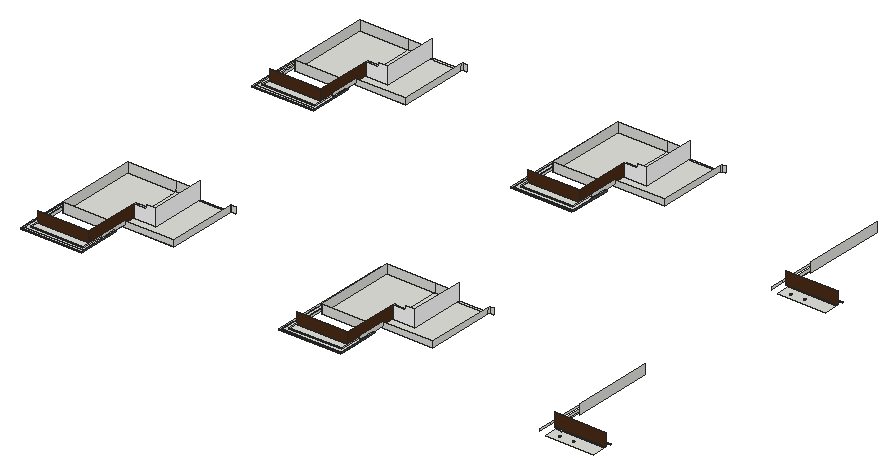
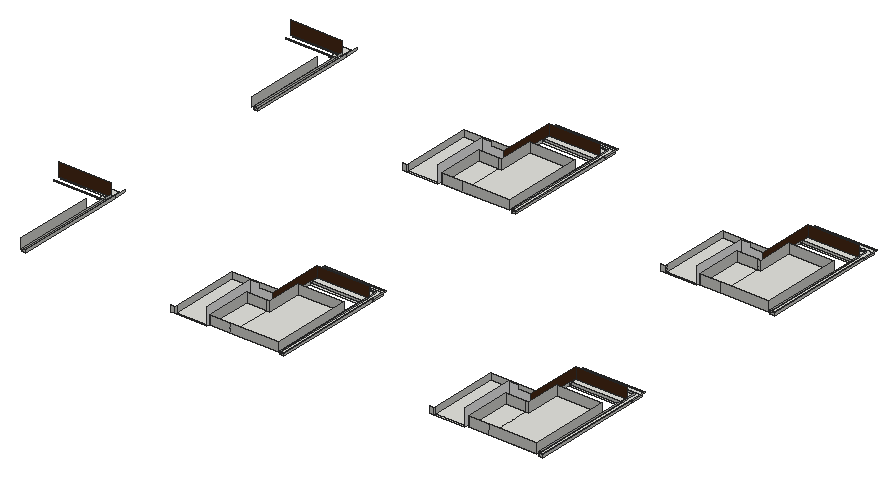
# SketchUp Ruby script. Lengths in inches.
U = 1.inch
M = Sketchup.active_model
def pt(a) = Geom::Point3d.new(a.map { |v| v * U })
def face(e, loops, mat)
  f = e.add_face(loops[0].map { |a| pt(a) })
  loops[1..].each { |l| e.add_face(l.map { |a| pt(a) }).erase! }
  f.material = f.back_material = mat if mat
  f
end
# faces: each face lists its corners as indices into pts; further lists are holes
def faces(e, pts, list, mat = nil) = list.each { |f| face(e, (f[0].is_a?(Array) ? f : [f]).map { |l| l.map { |i| pts[i] } }, mat) }
# xy, xz, yz: faces in a plane at the given z, y or x. An outline is a flat list of corners, or four numbers for a rectangle; further outlines are holes
def ring(l) = l.size == 4 ? [[l[0], l[1]], [l[2], l[1]], [l[2], l[3]], [l[0], l[3]]] : l.each_slice(2).to_a
def flat(e, list, mat, &to3) = list.each { |f| face(e, (f[0].is_a?(Array) ? f : [f]).map { |l| ring(l).map { |u, v| to3.(u, v) } }, mat) }
def xy(e, z, list, mat = nil) = flat(e, list, mat) { |x, y| [x, y, z] }
def xz(e, y, list, mat = nil) = flat(e, list, mat) { |x, z| [x, y, z] }
def yz(e, x, list, mat = nil) = flat(e, list, mat) { |y, z| [x, y, z] }
def lines(e, pts, list) = list.each { |a, b| e.add_line(pt(pts[a]), pt(pts[b])) }
# prism: a flat outline (further loops are holes) pulled along v
def prism(e, loops, v, mat = nil)
  f = face(e, loops, mat); d = Geom::Vector3d.new(v.map { |x| x * U })
  f.pushpull(f.normal.samedirection?(d) ? d.length : -d.length)
end
def box(e, o, s, mat = nil) = prism(e, [[o, [o[0] + s[0], o[1], o[2]], [o[0] + s[0], o[1] + s[1], o[2]], [o[0], o[1] + s[1], o[2]]]], [0, 0, s[2]], mat)
def at(x, y, z, deg = 0) = Geom::Transformation.translation(pt([x, y, z])) * Geom::Transformation.rotation(ORIGIN, Z_AXIS, deg.degrees)
def axes(o, x, y, z) = Geom::Transformation.new([*x, 0, *y, 0, *z, 0, *pt(o).to_a, 1])
def part(name) = M.definitions.add(name)
# library, detail: a bought-in or finely detailed component or shape, given as its bounding box
def library(name, o, s) = part(name).tap { |d| box(d.entities, o, s) }
def detail(e, o, s) = box(e.add_group.entities, o, s)
def put(e, d, t, mat = nil) = e.add_instance(d, t).tap { |i| i.material = mat if mat }
def group(e, t, mat = nil) = e.add_group.tap { |g| g.transformation = t; g.material = mat if mat }.entities
root = M.entities
M.materials.add("[Color M00]").color = [255, 255, 255]
M.materials.add("[Color M06]").color = [86, 86, 86]
M.materials.add("[Wood Veneer 01]").color = [76, 44, 23]
xy(root,257.1875,[[[2084.76,592.75,2251.32,636.6875],[2116.33,609.37,2117.03,609.46,2117.68,609.73,2118.23,610.15,2118.66,610.71,2118.93,611.36,2119.02,612.06,2118.93,612.75,2118.66,613.4,2118.23,613.96,2117.68,614.38,2117.03,614.65,2116.33,614.74,2115.64,614.65,2114.99,614.38,2114.43,613.96,2114.01,613.4,2113.74,612.75,2113.65,612.06,2113.74,611.36,2114.01,610.71,2114.43,610.15,2114.99,609.73,2115.64,609.46],[2164.33,609.37,2165.03,609.46,2165.68,609.73,2166.23,610.15,2166.66,610.71,2166.93,611.36,2167.02,612.06,2166.93,612.75,2166.66,613.4,2166.23,613.96,2165.68,614.38,2165.03,614.65,2164.33,614.74,2163.64,614.65,2162.99,614.38,2162.43,613.96,2162.01,613.4,2161.74,612.75,2161.65,612.06,2161.74,611.36,2162.01,610.71,2162.43,610.15,2162.99,609.73,2163.64,609.46],[2228.96,609.37,2229.65,609.46,2230.3,609.73,2230.86,610.15,2231.29,610.71,2231.55,611.36,2231.65,612.06,2231.55,612.75,2231.29,613.4,2230.86,613.96,2230.3,614.38,2229.65,614.65,2228.96,614.74,2228.26,614.65,2227.61,614.38,2227.06,613.96,2226.63,613.4,2226.36,612.75,2226.27,612.06,2226.36,611.36,2226.63,610.71,2227.06,610.15,2227.61,609.73,2228.26,609.46]],[2094.14,636.6875,2106.51,660.21],[[2084.76,1592.1,2251.32,1636.04],[2116.33,1608.72,2117.03,1608.8125,2117.68,1609.08,2118.23,1609.51,2118.66,1610.07,2118.93,1610.71,2119.02,1611.41,2118.93,1612.11,2118.66,1612.75,2118.23,1613.3125,2117.68,1613.74,2117.03,1614.01,2116.33,1614.1,2115.64,1614.01,2114.99,1613.74,2114.43,1613.3125,2114.01,1612.75,2113.74,1612.11,2113.65,1611.41,2113.74,1610.71,2114.01,1610.07,2114.43,1609.51,2114.99,1609.08,2115.64,1608.8125],[2164.33,1608.72,2165.03,1608.8125,2165.68,1609.08,2166.23,1609.51,2166.66,1610.07,2166.93,1610.71,2167.02,1611.41,2166.93,1612.11,2166.66,1612.75,2166.23,1613.3125,2165.68,1613.74,2165.03,1614.01,2164.33,1614.1,2163.64,1614.01,2162.99,1613.74,2162.43,1613.3125,2162.01,1612.75,2161.74,1612.11,2161.65,1611.41,2161.74,1610.71,2162.01,1610.07,2162.43,1609.51,2162.99,1609.08,2163.64,1608.8125],[2228.96,1608.72,2229.65,1608.8125,2230.3,1609.08,2230.86,1609.51,2231.29,1610.07,2231.55,1610.71,2231.65,1611.41,2231.55,1612.11,2231.29,1612.75,2230.86,1613.3125,2230.3,1613.74,2229.65,1614.01,2228.96,1614.1,2228.26,1614.01,2227.61,1613.74,2227.06,1613.3125,2226.63,1612.75,2226.36,1612.11,2226.27,1611.41,2226.36,1610.71,2226.63,1610.07,2227.06,1609.51,2227.61,1609.08,2228.26,1608.8125]],[2094.14,1636.04,2106.51,1659.57]])
xy(root,258.1875,[[294.47,639.17,471.68,662.52],[1187.0625,639.17,1364.27,662.52],[294.47,662.52,471.68,670.48],[1187.0625,662.52,1364.27,670.48],[304.78,733.75,462.15,733.75,462.15,854.49,471.68,854.49,471.68,1014.93,304.78,1014.93],
  [1197.375,733.75,1354.74,733.75,1354.74,854.49,1364.27,854.49,1364.27,1014.93,1197.375,1014.93],[471.68,776.62,655.66,776.62,655.66,1014.93,548.11,1014.93,548.11,832.12,471.68,832.12],[1364.27,776.62,1548.25,776.62,1548.25,1014.93,1440.7,1014.93,1440.7,832.12,1364.27,832.12],[471.68,854.49,542.11,1014.93],[1364.27,854.49,1434.7,1014.93],
  [548.11,1014.93,655.66,1021.31],[1440.7,1014.93,1548.25,1021.31],[294.47,1638.53,471.68,1661.875],[1187.0625,1638.53,1364.27,1661.875],[294.47,1661.875,471.68,1669.84],
  [1187.0625,1661.875,1364.27,1669.84],[304.78,1733.11,462.15,1733.11,462.15,1853.85,471.68,1853.85,471.68,2014.29,304.78,2014.29],[1197.375,1733.11,1354.74,1733.11,1354.74,1853.85,1364.27,1853.85,1364.27,2014.29,1197.375,2014.29],[471.68,1775.97,655.66,1775.97,655.66,2014.29,548.11,2014.29,548.11,1831.47,471.68,1831.47],[1364.27,1775.97,1548.25,1775.97,1548.25,2014.29,1440.7,2014.29,1440.7,1831.47,1364.27,1831.47],
  [471.68,1853.85,542.11,2014.29],[1364.27,1853.85,1434.7,2014.29],[548.11,2014.29,655.66,2020.66],[1440.7,2014.29,1548.25,2020.66]])
xy(root,265.6875,[[278.36,584.06,490.8,595.06],[1170.95,584.06,1383.39,595.06],[278.36,595.06,279.74,638.99],[279.74,595.06,279.74,1021.31,294.47,1021.31,294.47,607.33,475.29,607.33,475.29,706.17,484.3,706.17,484.3,595.06],[484.3,595.06,490.8,638.99],
  [1170.95,595.06,1172.33,638.99],[1172.33,595.06,1172.33,1021.31,1187.0625,1021.31,1187.0625,607.33,1367.875,607.33,1367.875,706.17,1376.89,706.17,1376.89,595.06],[1376.89,595.06,1383.39,638.99],[294.47,607.33,475.29,607.33,475.29,706.17,471.68,706.17,471.68,662.52,294.47,662.52],[1187.0625,607.33,1367.875,607.33,1367.875,706.17,1364.27,706.17,1364.27,662.52,1187.0625,662.52],
  [484.3,638.99,490.8,731.24],[1376.89,638.99,1383.39,731.24],[471.68,706.17,484.3,776.62],[1364.27,706.17,1376.89,776.62],[278.36,1583.41,490.8,1594.41],
  [1170.95,1583.41,1383.39,1594.41],[278.36,1594.41,279.74,1638.35],[279.74,1594.41,279.74,2020.66,294.47,2020.66,294.47,1606.6875,475.29,1606.6875,475.29,1705.53,484.3,1705.53,484.3,1594.41],[484.3,1594.41,490.8,1638.35],[1170.95,1594.41,1172.33,1638.35],
  [1172.33,1594.41,1172.33,2020.66,1187.0625,2020.66,1187.0625,1606.6875,1367.875,1606.6875,1367.875,1705.53,1376.89,1705.53,1376.89,1594.41],[1376.89,1594.41,1383.39,1638.35],[294.47,1606.6875,475.29,1606.6875,475.29,1705.53,471.68,1705.53,471.68,1661.875,294.47,1661.875],[1187.0625,1606.6875,1367.875,1606.6875,1367.875,1705.53,1364.27,1705.53,1364.27,1661.875,1187.0625,1661.875],[484.3,1638.35,490.8,1730.6],
  [1376.89,1638.35,1383.39,1730.6],[471.68,1705.53,484.3,1775.97],[1364.27,1705.53,1376.89,1775.97]])
xz(root,584.06,[[278.36,265.6875,490.8,269.375],[1170.95,265.6875,1383.39,269.375]],"[Color M06]")
xz(root,607.33,[[294.47,265.6875,475.29,269.375],[1187.0625,265.6875,1367.875,269.375]])
xz(root,636.86,[[2079.65,262.875,2256.86,307.5]],"[Wood Veneer 01]")
xz(root,638.99,[[278.36,265.6875,279.74,269.375],[1170.95,265.6875,1172.33,269.375]])
xz(root,639.17,[[294.47,258.1875,471.68,302.8125],[1187.0625,258.1875,1364.27,302.8125]],"[Wood Veneer 01]")
xz(root,660.21,[[2079.65,259.3125,2256.86,262.875]])
xz(root,662.52,[[294.47,258.1875,471.68,265.6875],[1187.0625,258.1875,1364.27,265.6875]])
xz(root,706.17,[[475.29,265.6875,484.3,269.375],[1367.875,265.6875,1376.89,269.375]])
xz(root,733.75,[[304.78,258.1875,462.15,291.125],[1197.375,258.1875,1354.74,291.125]])
xz(root,776.62,[[471.68,258.1875,471.68,265.6875,484.3,265.6875,484.3,279.25,655.66,279.25,655.66,258.1875],[1364.27,258.1875,1364.27,265.6875,1376.89,265.6875,1376.89,279.25,1548.25,279.25,1548.25,258.1875]])
xz(root,832.12,[[471.68,258.1875,548.11,258.1875,548.11,316.0625,518.11,316.0625,518.11,302.8125,471.68,302.8125],[1364.27,258.1875,1440.7,258.1875,1440.7,316.0625,1410.7,316.0625,1410.7,302.8125,1364.27,302.8125]],"[Color M00]")
xz(root,854.49,[[462.15,258.1875,471.68,291.125],[471.68,258.1875,542.11,291.125],[1354.74,258.1875,1364.27,291.125],[1364.27,258.1875,1434.7,291.125]])
xz(root,1014.93,[[304.78,258.1875,471.68,291.125],[471.68,258.1875,542.11,291.125],[1197.375,258.1875,1364.27,291.125],[1364.27,258.1875,1434.7,291.125]])
xz(root,1019,[[2064.92,262.875,2079.65,270.375]])
xz(root,1021.31,[[279.74,258.1875,294.47,265.6875],[655.66,258.1875,671.36,279.25],[1172.33,258.1875,1187.0625,265.6875],[1548.25,258.1875,1563.95,279.25],[279.74,265.6875,294.47,269.375],
  [1172.33,265.6875,1187.0625,269.375]])
xz(root,1583.41,[[278.36,265.6875,490.8,269.375],[1170.95,265.6875,1383.39,269.375]],"[Color M06]")
xz(root,1606.6875,[[294.47,265.6875,475.29,269.375],[1187.0625,265.6875,1367.875,269.375]])
xz(root,1636.22,[[2079.65,262.875,2256.86,307.5]],"[Wood Veneer 01]")
xz(root,1638.35,[[278.36,265.6875,279.74,269.375],[1170.95,265.6875,1172.33,269.375]])
xz(root,1638.53,[[294.47,258.1875,471.68,302.8125],[1187.0625,258.1875,1364.27,302.8125]],"[Wood Veneer 01]")
xz(root,1659.57,[[2079.65,259.3125,2256.86,262.875]])
xz(root,1661.875,[[294.47,258.1875,471.68,265.6875],[1187.0625,258.1875,1364.27,265.6875]])
xz(root,1705.53,[[475.29,265.6875,484.3,269.375],[1367.875,265.6875,1376.89,269.375]])
xz(root,1733.11,[[304.78,258.1875,462.15,291.125],[1197.375,258.1875,1354.74,291.125]])
xz(root,1775.97,[[471.68,258.1875,471.68,265.6875,484.3,265.6875,484.3,279.25,655.66,279.25,655.66,258.1875],[1364.27,258.1875,1364.27,265.6875,1376.89,265.6875,1376.89,279.25,1548.25,279.25,1548.25,258.1875]])
xz(root,1831.47,[[471.68,258.1875,548.11,258.1875,548.11,316.0625,518.11,316.0625,518.11,302.8125,471.68,302.8125],[1364.27,258.1875,1440.7,258.1875,1440.7,316.0625,1410.7,316.0625,1410.7,302.8125,1364.27,302.8125]],"[Color M00]")
xz(root,1853.85,[[462.15,258.1875,471.68,291.125],[471.68,258.1875,542.11,291.125],[1354.74,258.1875,1364.27,291.125],[1364.27,258.1875,1434.7,291.125]])
xz(root,2014.29,[[304.78,258.1875,471.68,291.125],[471.68,258.1875,542.11,291.125],[1197.375,258.1875,1364.27,291.125],[1364.27,258.1875,1434.7,291.125]])
xz(root,2018.36,[[2064.92,262.875,2079.65,270.375]])
xz(root,2020.66,[[279.74,258.1875,294.47,265.6875],[655.66,258.1875,671.36,279.25],[1172.33,258.1875,1187.0625,265.6875],[1548.25,258.1875,1563.95,279.25],[279.74,265.6875,294.47,269.375],
  [1172.33,265.6875,1187.0625,269.375]])
yz(root,278.36,[[584.06,265.6875,638.99,269.375],[1583.41,265.6875,1638.35,269.375]])
yz(root,279.74,[[595.06,258.1875,638.99,265.6875],[638.99,258.1875,1021.31,265.6875],[1594.41,258.1875,1638.35,265.6875],[1638.35,258.1875,2020.66,265.6875],[638.99,265.6875,1021.31,269.375],
  [1638.35,265.6875,2020.66,269.375]])
yz(root,294.47,[[639.17,258.1875,662.52,265.6875],[662.52,258.1875,670.48,265.6875],[670.48,258.1875,1014.93,265.6875],[1014.93,258.1875,1021.31,265.6875],[1638.53,258.1875,1661.875,265.6875],
  [1661.875,258.1875,1669.84,265.6875],[1669.84,258.1875,2014.29,265.6875],[2014.29,258.1875,2020.66,265.6875],[607.33,265.6875,639.17,269.375],[639.17,265.6875,662.52,269.375],
  [662.52,265.6875,670.48,269.375],[670.48,265.6875,1014.93,269.375],[1014.93,265.6875,1021.31,269.375],[1606.6875,265.6875,1638.53,269.375],[1638.53,265.6875,1661.875,269.375],
  [1661.875,265.6875,1669.84,269.375],[1669.84,265.6875,2014.29,269.375],[2014.29,265.6875,2020.66,269.375]])
yz(root,304.78,[[733.75,258.1875,1014.93,291.125],[1733.11,258.1875,2014.29,291.125]])
yz(root,462.15,[[733.75,258.1875,854.49,291.125],[1733.11,258.1875,1853.85,291.125]])
yz(root,471.68,[[639.17,258.1875,662.52,265.6875],[662.52,258.1875,670.48,265.6875],[670.48,258.1875,738.06,265.6875],[738.06,258.1875,776.62,265.6875],[1638.53,258.1875,1661.875,265.6875],
  [1661.875,258.1875,1669.84,265.6875],[1669.84,258.1875,1737.41,265.6875],[1737.41,258.1875,1775.97,265.6875]])
yz(root,471.68,[[776.62,258.1875,832.12,258.1875,832.12,302.8125,639.17,302.8125,639.17,265.6875,776.62,265.6875],[1775.97,258.1875,1831.47,258.1875,1831.47,302.8125,1638.53,302.8125,1638.53,265.6875,1775.97,265.6875]],"[Wood Veneer 01]")
yz(root,475.29,[[607.33,265.6875,706.17,269.375],[1606.6875,265.6875,1705.53,269.375]])
yz(root,484.3,[[731.24,265.6875,731.24,269.375,676.67,269.375,676.67,279.25,776.62,279.25,776.62,265.6875],[706.17,265.6875,731.24,269.375],[1730.6,265.6875,1730.6,269.375,1676.03,269.375,1676.03,279.25,1775.97,279.25,1775.97,265.6875],[1705.53,265.6875,1730.6,269.375]])
yz(root,490.8,[[584.06,265.6875,731.24,269.375],[1583.41,265.6875,1730.6,269.375]],"[Color M06]")
yz(root,542.11,[[854.49,258.1875,1014.93,291.125],[1853.85,258.1875,2014.29,291.125]])
yz(root,548.11,[[832.12,258.1875,1021.31,316.0625],[1831.47,258.1875,2020.66,316.0625]],"[Color M00]")
yz(root,655.66,[[776.62,258.1875,1014.93,279.25],[1014.93,258.1875,1021.31,279.25],[1775.97,258.1875,2014.29,279.25],[2014.29,258.1875,2020.66,279.25]])
yz(root,1170.95,[[584.06,265.6875,638.99,269.375],[1583.41,265.6875,1638.35,269.375]])
yz(root,1172.33,[[595.06,258.1875,638.99,265.6875],[638.99,258.1875,1021.31,265.6875],[1594.41,258.1875,1638.35,265.6875],[1638.35,258.1875,2020.66,265.6875],[638.99,265.6875,1021.31,269.375],
  [1638.35,265.6875,2020.66,269.375]])
yz(root,1187.0625,[[639.17,258.1875,662.52,265.6875],[662.52,258.1875,670.48,265.6875],[670.48,258.1875,1014.93,265.6875],[1014.93,258.1875,1021.31,265.6875],[1638.53,258.1875,1661.875,265.6875],
  [1661.875,258.1875,1669.84,265.6875],[1669.84,258.1875,2014.29,265.6875],[2014.29,258.1875,2020.66,265.6875],[607.33,265.6875,639.17,269.375],[639.17,265.6875,662.52,269.375],
  [662.52,265.6875,670.48,269.375],[670.48,265.6875,1014.93,269.375],[1014.93,265.6875,1021.31,269.375],[1606.6875,265.6875,1638.53,269.375],[1638.53,265.6875,1661.875,269.375],
  [1661.875,265.6875,1669.84,269.375],[1669.84,265.6875,2014.29,269.375],[2014.29,265.6875,2020.66,269.375]])
yz(root,1197.375,[[733.75,258.1875,1014.93,291.125],[1733.11,258.1875,2014.29,291.125]])
yz(root,1354.74,[[733.75,258.1875,854.49,291.125],[1733.11,258.1875,1853.85,291.125]])
yz(root,1364.27,[[639.17,258.1875,662.52,265.6875],[662.52,258.1875,670.48,265.6875],[670.48,258.1875,738.06,265.6875],[738.06,258.1875,776.62,265.6875],[1638.53,258.1875,1661.875,265.6875],
  [1661.875,258.1875,1669.84,265.6875],[1669.84,258.1875,1737.41,265.6875],[1737.41,258.1875,1775.97,265.6875]])
yz(root,1364.27,[[776.62,258.1875,832.12,258.1875,832.12,302.8125,639.17,302.8125,639.17,265.6875,776.62,265.6875],[1775.97,258.1875,1831.47,258.1875,1831.47,302.8125,1638.53,302.8125,1638.53,265.6875,1775.97,265.6875]],"[Wood Veneer 01]")
yz(root,1367.875,[[607.33,265.6875,706.17,269.375],[1606.6875,265.6875,1705.53,269.375]])
yz(root,1376.89,[[731.24,265.6875,731.24,269.375,676.67,269.375,676.67,279.25,776.62,279.25,776.62,265.6875],[706.17,265.6875,731.24,269.375],[1730.6,265.6875,1730.6,269.375,1676.03,269.375,1676.03,279.25,1775.97,279.25,1775.97,265.6875],[1705.53,265.6875,1730.6,269.375]])
yz(root,1383.39,[[584.06,265.6875,731.24,269.375],[1583.41,265.6875,1730.6,269.375]],"[Color M06]")
yz(root,1434.7,[[854.49,258.1875,1014.93,291.125],[1853.85,258.1875,2014.29,291.125]])
yz(root,1440.7,[[832.12,258.1875,1021.31,316.0625],[1831.47,258.1875,2020.66,316.0625]],"[Color M00]")
yz(root,1548.25,[[776.62,258.1875,1014.93,279.25],[1014.93,258.1875,1021.31,279.25],[1775.97,258.1875,2014.29,279.25],[2014.29,258.1875,2020.66,279.25]])
yz(root,2064.92,[[592.75,262.875,636.6875,270.375],[636.6875,262.875,1019,270.375],[1592.1,262.875,1636.04,270.375],[1636.04,262.875,2018.36,270.375]])
yz(root,2079.65,[[660.21,259.3125,1012.63,262.875],[1659.57,259.3125,2011.98,262.875],[636.86,262.875,660.21,270.375],[660.21,262.875,668.18,270.375],[668.18,262.875,1012.63,270.375],
  [1012.63,262.875,1019,270.375],[1636.22,262.875,1659.57,270.375],[1659.57,262.875,1667.53,270.375],[1667.53,262.875,2011.98,270.375],[2011.98,262.875,2018.36,270.375]])
yz(root,2089.96,[[731.45,262.875,1012.63,295.8125],[1730.8,262.875,2011.98,295.8125]])
p = [[2116.33,609.37,257.1875],[2115.64,609.46,257.1875],[2115.64,609.46,257.6875],[2116.33,609.37,257.6875],[2117.03,609.46,257.1875],[2117.03,609.46,257.6875],
  [2164.33,609.37,257.1875],[2163.64,609.46,257.1875],[2163.64,609.46,257.8125],[2164.33,609.37,257.8125],[2165.03,609.46,257.1875],[2165.03,609.46,257.8125],
  [2114.99,609.73,257.1875],[2114.99,609.73,257.6875],[2117.68,609.73,257.1875],[2117.68,609.73,257.6875],[2162.99,609.73,257.1875],[2162.99,609.73,257.8125],
  [2165.68,609.73,257.1875],[2165.68,609.73,257.8125],[2114.43,610.15,257.1875],[2114.43,610.15,257.6875],[2118.23,610.15,257.1875],[2118.23,610.15,257.6875],
  [2162.43,610.15,257.1875],[2162.43,610.15,257.8125],[2166.23,610.15,257.1875],[2166.23,610.15,257.8125],[2114.01,610.71,257.1875],[2114.01,610.71,257.6875],
  [2118.66,610.71,257.1875],[2118.66,610.71,257.6875],[2162.01,610.71,257.1875],[2162.01,610.71,257.8125],[2166.66,610.71,257.1875],[2166.66,610.71,257.8125],
  [2113.74,611.36,257.1875],[2113.74,611.36,257.6875],[2118.93,611.36,257.1875],[2118.93,611.36,257.6875],[2161.74,611.36,257.1875],[2161.74,611.36,257.8125],
  [2166.93,611.36,257.1875],[2166.93,611.36,257.8125],[2113.65,612.06,257.1875],[2113.65,612.06,257.6875],[2119.02,612.06,257.1875],[2119.02,612.06,257.6875],
  [2161.65,612.06,257.1875],[2161.65,612.06,257.8125],[2167.02,612.06,257.1875],[2167.02,612.06,257.8125],[2113.74,612.75,257.1875],[2113.74,612.75,257.6875],
  [2118.93,612.75,257.1875],[2118.93,612.75,257.6875],[2161.74,612.75,257.1875],[2161.74,612.75,257.8125],[2166.93,612.75,257.1875],[2166.93,612.75,257.8125],
  [2114.01,613.4,257.1875],[2114.01,613.4,257.6875],[2118.66,613.4,257.1875],[2118.66,613.4,257.6875],[2162.01,613.4,257.1875],[2162.01,613.4,257.8125],
  [2166.66,613.4,257.1875],[2166.66,613.4,257.8125],[2114.43,613.96,257.1875],[2114.43,613.96,257.6875],[2118.23,613.96,257.1875],[2118.23,613.96,257.6875],
  [2162.43,613.96,257.1875],[2162.43,613.96,257.8125],[2166.23,613.96,257.1875],[2166.23,613.96,257.8125],[2114.99,614.38,257.1875],[2114.99,614.38,257.6875],
  [2117.68,614.38,257.1875],[2117.68,614.38,257.6875],[2162.99,614.38,257.1875],[2162.99,614.38,257.8125],[2165.68,614.38,257.1875],[2165.68,614.38,257.8125],
  [2115.64,614.65,257.1875],[2115.64,614.65,257.6875],[2117.03,614.65,257.1875],[2117.03,614.65,257.6875],[2163.64,614.65,257.1875],[2163.64,614.65,257.8125],
  [2165.03,614.65,257.1875],[2165.03,614.65,257.8125],[2116.33,614.74,257.1875],[2116.33,614.74,257.6875],[2164.33,614.74,257.1875],[2164.33,614.74,257.8125],
  [2116.33,1608.72,257.1875],[2115.64,1608.8125,257.1875],[2115.64,1608.8125,257.6875],[2116.33,1608.72,257.6875],[2117.03,1608.8125,257.1875],[2117.03,1608.8125,257.6875],
  [2164.33,1608.72,257.1875],[2163.64,1608.8125,257.1875],[2163.64,1608.8125,257.8125],[2164.33,1608.72,257.8125],[2165.03,1608.8125,257.1875],[2165.03,1608.8125,257.8125],
  [2114.99,1609.08,257.1875],[2114.99,1609.08,257.6875],[2117.68,1609.08,257.1875],[2117.68,1609.08,257.6875],[2162.99,1609.08,257.1875],[2162.99,1609.08,257.8125],
  [2165.68,1609.08,257.1875],[2165.68,1609.08,257.8125],[2114.43,1609.51,257.1875],[2114.43,1609.51,257.6875],[2118.23,1609.51,257.1875],[2118.23,1609.51,257.6875],
  [2162.43,1609.51,257.1875],[2162.43,1609.51,257.8125],[2166.23,1609.51,257.1875],[2166.23,1609.51,257.8125],[2114.01,1610.07,257.1875],[2114.01,1610.07,257.6875],
  [2118.66,1610.07,257.1875],[2118.66,1610.07,257.6875],[2162.01,1610.07,257.1875],[2162.01,1610.07,257.8125],[2166.66,1610.07,257.1875],[2166.66,1610.07,257.8125],
  [2113.74,1610.71,257.1875],[2113.74,1610.71,257.6875],[2118.93,1610.71,257.1875],[2118.93,1610.71,257.6875],[2161.74,1610.71,257.1875],[2161.74,1610.71,257.8125],
  [2166.93,1610.71,257.1875],[2166.93,1610.71,257.8125],[2113.65,1611.41,257.1875],[2113.65,1611.41,257.6875],[2119.02,1611.41,257.1875],[2119.02,1611.41,257.6875],
  [2161.65,1611.41,257.1875],[2161.65,1611.41,257.8125],[2167.02,1611.41,257.1875],[2167.02,1611.41,257.8125],[2113.74,1612.11,257.1875],[2113.74,1612.11,257.6875],
  [2118.93,1612.11,257.1875],[2118.93,1612.11,257.6875],[2161.74,1612.11,257.1875],[2161.74,1612.11,257.8125],[2166.93,1612.11,257.1875],[2166.93,1612.11,257.8125],
  [2114.01,1612.75,257.1875],[2114.01,1612.75,257.6875],[2118.66,1612.75,257.1875],[2118.66,1612.75,257.6875],[2162.01,1612.75,257.1875],[2162.01,1612.75,257.8125],
  [2166.66,1612.75,257.1875],[2166.66,1612.75,257.8125],[2114.43,1613.3125,257.1875],[2114.43,1613.3125,257.6875],[2118.23,1613.3125,257.1875],[2118.23,1613.3125,257.6875],
  [2162.43,1613.3125,257.1875],[2162.43,1613.3125,257.8125],[2166.23,1613.3125,257.1875],[2166.23,1613.3125,257.8125],[2114.99,1613.74,257.1875],[2114.99,1613.74,257.6875],
  [2117.68,1613.74,257.1875],[2117.68,1613.74,257.6875],[2162.99,1613.74,257.1875],[2162.99,1613.74,257.8125],[2165.68,1613.74,257.1875],[2165.68,1613.74,257.8125],
  [2115.64,1614.01,257.1875],[2115.64,1614.01,257.6875],[2117.03,1614.01,257.1875],[2117.03,1614.01,257.6875],[2163.64,1614.01,257.1875],[2163.64,1614.01,257.8125],
  [2165.03,1614.01,257.1875],[2165.03,1614.01,257.8125],[2116.33,1614.1,257.1875],[2116.33,1614.1,257.6875],[2164.33,1614.1,257.1875],[2164.33,1614.1,257.8125],
  [471.68,776.62,265.6875],[471.68,776.62,277.5],[1364.27,776.62,265.6875],[1364.27,776.62,277.5],[471.68,1775.97,265.6875],[471.68,1775.97,277.5],
  [1364.27,1775.97,265.6875],[1364.27,1775.97,277.5]]
faces(root,p,[[0,1,2,3],[4,0,3,5],[6,7,8,9],[10,6,9,11],[1,12,13,2],[14,4,5,15],[7,16,17,8],[18,10,11,19],
  [12,20,21,13],[22,14,15,23],[16,24,25,17],[26,18,19,27],[20,28,29,21],[30,22,23,31],[24,32,33,25],[34,26,27,35],
  [28,36,37,29],[38,30,31,39],[32,40,41,33],[42,34,35,43],[36,44,45,37],[46,38,39,47],[40,48,49,41],[50,42,43,51],
  [44,52,53,45],[54,46,47,55],[48,56,57,49],[58,50,51,59],[52,60,61,53],[62,54,55,63],[56,64,65,57],[66,58,59,67],
  [60,68,69,61],[70,62,63,71],[64,72,73,65],[74,66,67,75],[68,76,77,69],[78,70,71,79],[72,80,81,73],[82,74,75,83],
  [76,84,85,77],[86,78,79,87],[80,88,89,81],[90,82,83,91],[84,92,93,85],[92,86,87,93],[88,94,95,89],[94,90,91,95],
  [96,97,98,99],[100,96,99,101],[102,103,104,105],[106,102,105,107],[97,108,109,98],[110,100,101,111],[103,112,113,104],[114,106,107,115],
  [108,116,117,109],[118,110,111,119],[112,120,121,113],[122,114,115,123],[116,124,125,117],[126,118,119,127],[120,128,129,121],[130,122,123,131],
  [124,132,133,125],[134,126,127,135],[128,136,137,129],[138,130,131,139],[132,140,141,133],[142,134,135,143],[136,144,145,137],[146,138,139,147],
  [140,148,149,141],[150,142,143,151],[144,152,153,145],[154,146,147,155],[148,156,157,149],[158,150,151,159],[152,160,161,153],[162,154,155,163],
  [156,164,165,157],[166,158,159,167],[160,168,169,161],[170,162,163,171],[164,172,173,165],[174,166,167,175],[168,176,177,169],[178,170,171,179],
  [172,180,181,173],[182,174,175,183],[176,184,185,177],[186,178,179,187],[180,188,189,181],[188,182,183,189],[184,190,191,185],[190,186,187,191]])
lines(root,p,[[192,193],[194,195],[196,197],[198,199]])
